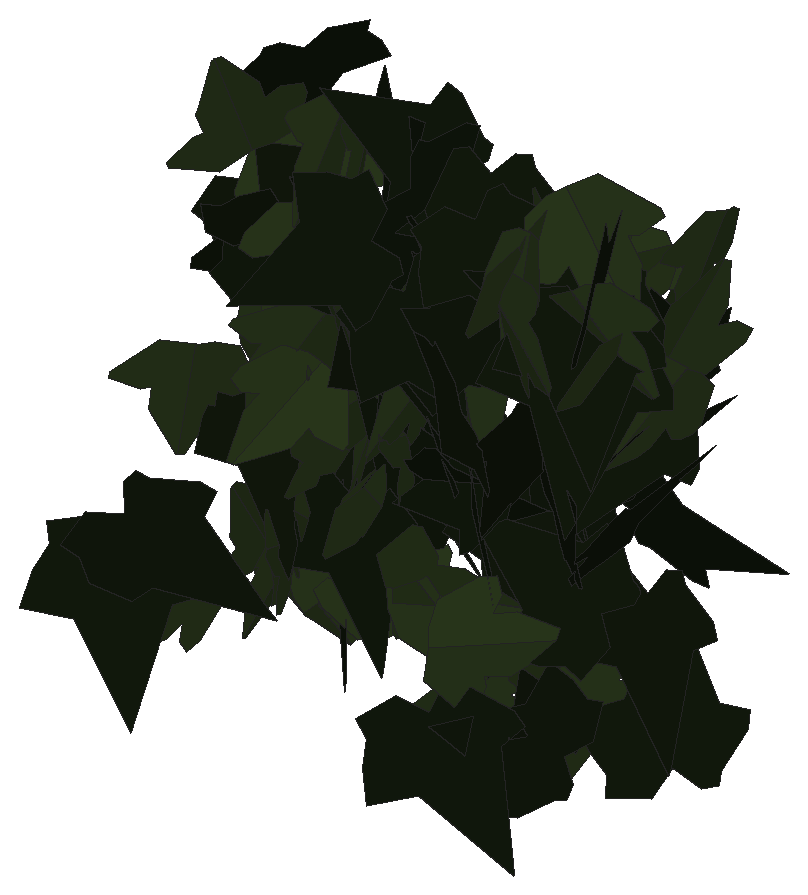
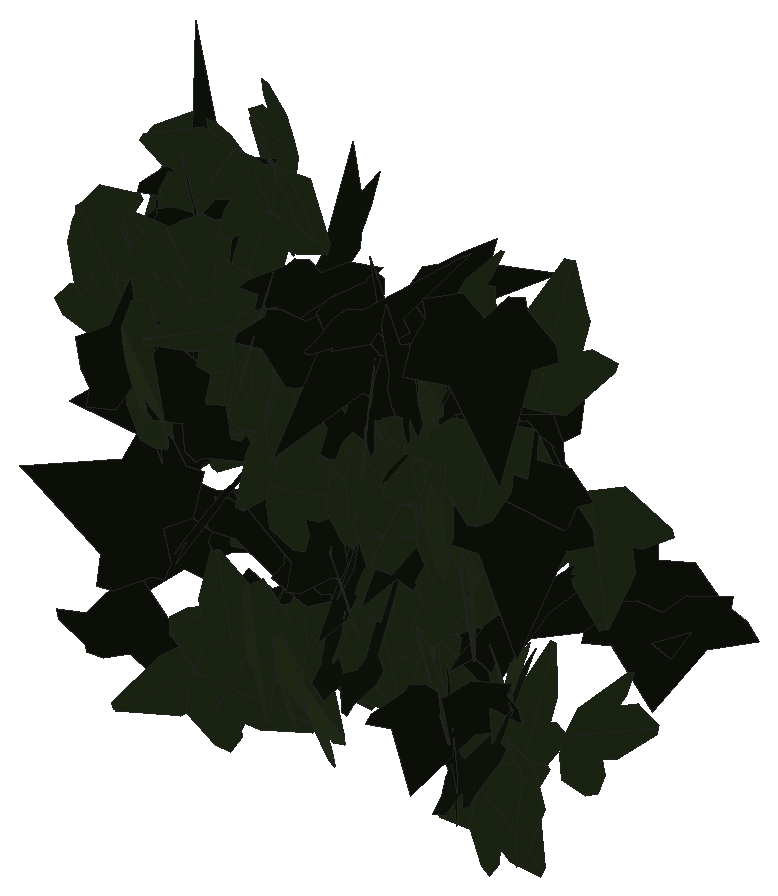
# SketchUp Ruby script. Lengths in inches.
U = 1.inch
M = Sketchup.active_model
def pt(a) = Geom::Point3d.new(a.map { |v| v * U })
def face(e, loops, mat)
  f = e.add_face(loops[0].map { |a| pt(a) })
  loops[1..].each { |l| e.add_face(l.map { |a| pt(a) }).erase! }
  f.material = f.back_material = mat if mat
  f
end
# faces: each face lists its corners as indices into pts; further lists are holes
def faces(e, pts, list, mat = nil) = list.each { |f| face(e, (f[0].is_a?(Array) ? f : [f]).map { |l| l.map { |i| pts[i] } }, mat) }
# xy, xz, yz: faces in a plane at the given z, y or x. An outline is a flat list of corners, or four numbers for a rectangle; further outlines are holes
def ring(l) = l.size == 4 ? [[l[0], l[1]], [l[2], l[1]], [l[2], l[3]], [l[0], l[3]]] : l.each_slice(2).to_a
def flat(e, list, mat, &to3) = list.each { |f| face(e, (f[0].is_a?(Array) ? f : [f]).map { |l| ring(l).map { |u, v| to3.(u, v) } }, mat) }
def xy(e, z, list, mat = nil) = flat(e, list, mat) { |x, y| [x, y, z] }
def xz(e, y, list, mat = nil) = flat(e, list, mat) { |x, z| [x, y, z] }
def yz(e, x, list, mat = nil) = flat(e, list, mat) { |y, z| [x, y, z] }
def lines(e, pts, list) = list.each { |a, b| e.add_line(pt(pts[a]), pt(pts[b])) }
# prism: a flat outline (further loops are holes) pulled along v
def prism(e, loops, v, mat = nil)
  f = face(e, loops, mat); d = Geom::Vector3d.new(v.map { |x| x * U })
  f.pushpull(f.normal.samedirection?(d) ? d.length : -d.length)
end
def box(e, o, s, mat = nil) = prism(e, [[o, [o[0] + s[0], o[1], o[2]], [o[0] + s[0], o[1] + s[1], o[2]], [o[0], o[1] + s[1], o[2]]]], [0, 0, s[2]], mat)
def at(x, y, z, deg = 0) = Geom::Transformation.translation(pt([x, y, z])) * Geom::Transformation.rotation(ORIGIN, Z_AXIS, deg.degrees)
def axes(o, x, y, z) = Geom::Transformation.new([*x, 0, *y, 0, *z, 0, *pt(o).to_a, 1])
def part(name) = M.definitions.add(name)
# library, detail: a bought-in or finely detailed component or shape, given as its bounding box
def library(name, o, s) = part(name).tap { |d| box(d.entities, o, s) }
def detail(e, o, s) = box(e.add_group.entities, o, s)
def put(e, d, t, mat = nil) = e.add_instance(d, t).tap { |i| i.material = mat if mat }
def group(e, t, mat = nil) = e.add_group.tap { |g| g.transformation = t; g.material = mat if mat }.entities
root = M.entities
M.materials.add("efeu1").color = [18, 25, 13]
M.materials.add("efeu2").color = [43, 57, 29]
c1 = part("ivyleaf_9")
p = [[1.54,2.16,1.25],[1.36,2.04,1.19],[-0.21,0.99,0.68],[-0.71,1.11,0.82],[-0.85,0.86,0.67],[-0.8,0.17,0.21],
  [-0.9,-0.01,0.1],[-0.67,-0.16,-0.02],[-0.08,-0.08,-0.05],[-0.03,-0.6,-0.4],[0.65,-0.88,-0.66],[0.83,-0.6,-0.49],
  [1.29,-0.42,-0.43],[1.8125,-0.07,-0.26],[1.21,0.44,0.15]]
faces(c1.entities,p,[[0,1,2,3,4,5,6,7,8,9,10,11,12,13,14]],"efeu1")
c2 = part("ivyleaf_10")
p = [[0,0.5,-0.03],[-0.0625,2.02,-0.43],[-0.19,2.01,-0.46],[-0.54,1.05,-0.29],[-0.52,0.625,-0.18],[-0.83,0.76,-0.28],
  [-1.16,0.64,-0.33],[-1.15,0.33,-0.24],[-0.77,-0.39,0.02],[-0.3,-0.51,0.16],[0.04,-0.48,0.23],[-0.02,2.01,-0.4375],
  [-0.06,2.01,-0.43],[0.04,-0.49,0.23],[0.67,-0.49,0.14],[1.38,0.36,-0.2],[1.375,0.51,-0.24],[0.81,0.65,-0.19],
  [0.62,0.59,-0.15],[0.6,1.09,-0.28],[0.5,1.23,-0.31]]
faces(c2.entities,p,[[0,1,2,3,4,5,6,7,8,9,10],[11,12,0,13,14,15,16,17,18,19,20]],"efeu2")
put(root,c1,axes([524.83,131.26,166.07],[-0.33768,-0.70628,-0.39631],[0.18411,0.35119,-0.78275],[0.78867,-0.38439,0.01304]))
put(root,c1,axes([530.67,131.73,170.2],[-0.07037,-0.33618,0.8001],[0.17324,-0.79201,-0.31754],[0.85039,0.13353,0.1309]))
put(root,c1,axes([525.15,131.12,166.79],[-0.00324,-0.09918,-0.87578],[0.39129,0.78459,-0.0903],[0.78976,-0.38914,0.04115]))
put(root,c2,axes([531.55,131.88,171.93],[-0.12147,0.13012,-0.78485],[0.54193,-0.56772,-0.17799],[-0.58244,-0.55537,-0.00193]))
put(root,c1,axes([530.2,131.6875,165.03],[-0.16384,-0.49695,-0.6787],[0.3544,0.58631,-0.51485],[0.76288,-0.3791,0.09342]))
put(root,c2,axes([530.38,131.99,166.21],[0.0291,-0.18103,-0.81104],[0.58754,0.57838,-0.10802],[0.58766,-0.5693,0.14816]))
put(root,c2,axes([524.8125,133.125,164.82],[-0.15719,-0.20614,0.77495],[0.12655,-0.78618,-0.18346],[0.79185,0.08473,0.18315]))
put(root,c1,axes([527.77,133.2,171.31],[-0.42129,-0.39468,0.56978],[-0.37791,-0.42814,-0.57599],[0.58103,-0.56464,0.03849]))
put(root,c1,axes([532.14,132.8125,171.72],[-0.38102,-0.63351,-0.36322],[0.22429,0.28837,-0.73823],[0.69495,-0.4404,0.03911]))
put(root,c1,axes([531.28,133.14,168.17],[-0.03344,-0.04847,0.86819],[0.28188,-0.82252,-0.03507],[0.82259,0.27988,0.04731]))
put(root,c2,axes([530.8125,132.92,172.19],[0.68256,-0.389,0.246],[0.21069,-0.12712,-0.7856],[0.4092,0.71431,-0.00584]))
put(root,c1,axes([531.3,133.21,164.18],[-0.08881,-0.05871,0.77051],[-0.61522,-0.46393,-0.10626],[0.46758,-0.62156,0.00653]))
put(root,c1,axes([532,133.07,171.17],[-0.54813,-0.70434,-0.32675],[0.20045,0.25805,-0.89249],[0.75012,-0.58363,-0.00027]))
put(root,c2,axes([532.25,132.74,171.99],[-0.66193,-0.01059,-0.40762],[0.40749,0.01078,-0.66201],[0.01466,-0.7773,-0.00363]))
put(root,c1,axes([531.94,133.12,171.56],[0.0001,0.50919,0.71944],[-0.06815,-0.71728,0.50767],[0.87876,-0.05568,0.03929]))
put(root,c2,axes([524.84,132.94,168.43],[-0.56624,-0.593,0.10866],[-0.06735,-0.08591,-0.81986],[0.5991,-0.57014,0.01053]))
put(root,c2,axes([532.52,132.99,171.28],[0.07296,-0.88071,-0.02433],[-0.00149,0.02429,-0.88373],[0.88104,0.07297,0.00052]))
put(root,c1,axes([531.25,132.96,169.81],[-0.09911,0.68835,-0.5205],[0.08396,-0.51374,-0.69541],[-0.85889,-0.12965,-0.00792]))
put(root,c2,axes([526.66,133.17,168.63],[0.51564,0.31871,-0.46657],[-0.39582,-0.24702,-0.60618],[-0.40322,0.65004,-0.0016]))
put(root,c1,axes([529.7,133.49,167.01],[-0.13232,0.06257,0.84388],[0.09722,-0.84735,0.07807],[0.84059,0.10785,0.1238]))
put(root,c2,axes([526.64,133.34,169.4],[-0.35373,-0.58412,0.4179],[-0.2198,-0.35544,-0.68287],[0.68375,-0.41644,-0.00333]))
put(root,c2,axes([528.72,133.08,165.93],[-0.14963,-0.09225,0.88799],[0.82092,0.33964,0.17361],[-0.35087,0.834,0.02751]))
put(root,c2,axes([527.73,132.95,169.95],[-0.02166,0.01381,0.77347],[-0.71103,0.30446,-0.02534],[-0.30475,-0.71135,0.00417]))
put(root,c2,axes([529.73,132.97,164.72],[-0.47195,-0.41579,-0.57038],[0.45046,0.35082,-0.62846],[0.54342,-0.65192,0.02559]))
put(root,c2,axes([529.01,133.25,165.9],[-0.6294,-0.14357,-0.40165],[0.40387,0.02971,-0.6435],[0.13721,-0.74605,0.05167]))
put(root,c1,axes([530.11,133.28,168.2],[-0.60442,0.37288,0.29163],[-0.24716,0.1548,-0.71018],[-0.40373,-0.653,-0.00182]))
put(root,c2,axes([526.48,133.5,170.88],[0.57668,0.38275,-0.24351],[-0.20508,-0.13135,-0.69213],[-0.40465,0.61205,0.00375]))
put(root,c2,axes([525.72,133.89,165.36],[-0.36296,0.24349,0.72411],[0.49871,-0.53178,0.42879],[0.57872,0.61097,0.08463]))
put(root,c2,axes([528.16,134.09,168.91],[-0.0036,-0.27996,0.77289],[0.25579,-0.73491,-0.26501],[0.78122,0.23933,0.09033]))
put(root,c1,axes([532.14,132.97,167.89],[-0.10416,0.73094,-0.26665],[-0.03631,0.26417,0.73832],[0.77721,0.1103,-0.00124]))
put(root,c1,axes([531.5,133.83,171.625],[-0.46135,-0.61749,-0.21894],[0.13553,0.17203,-0.77078],[0.64098,-0.48081,0.00539]))
put(root,c2,axes([525.33,133.77,168.81],[-0.05503,0.04318,-0.72069],[0.6025,-0.39551,-0.06971],[-0.39781,-0.60498,-0.00587]))
put(root,c1,axes([531.53,133.74,166.39],[-0.56293,-0.4876,-0.29346],[-0.19672,-0.22061,0.7439],[-0.53402,0.59526,0.03531]))
put(root,c1,axes([528.83,133.59,167.47],[0.55109,0.18256,-0.49055],[0.45821,0.17604,0.58028],[0.253,-0.71649,0.01758]))
put(root,c2,axes([530.61,133.29,171.99],[-0.19029,-0.7711,-0.50217],[0.13692,0.48336,-0.7941],[0.90996,-0.23398,0.01447]))
put(root,c1,axes([527.1875,134.3,169.17],[0.45596,-0.43502,-0.60219],[0.43981,-0.41136,0.63018],[-0.5987,-0.63349,0.00432]))
put(root,c2,axes([527.77,134.14,167.73],[-0.37409,0.23327,0.68753],[0.41937,-0.56192,0.41884],[0.59265,0.54487,0.1376]))
put(root,c2,axes([529.6,134.08,165.1],[0.27593,-0.73905,0.40423],[0.18018,-0.36374,-0.78801],[0.82288,0.32747,0.037]))
put(root,c1,axes([527.06,133.84,166.47],[-0.45072,-0.26509,-0.65886],[0.59257,0.28975,-0.52194],[0.39145,-0.74384,0.03149]))
put(root,c2,axes([526.52,134.19,167.12],[-0.24711,-0.41663,-0.55415],[-0.18121,-0.52903,0.47855],[-0.66919,0.2971,0.07504]))
put(root,c1,axes([528.28,133.55,170.42],[0.15786,-0.60152,-0.6506],[0.00209,0.6611,-0.61071],[0.88606,0.10561,0.11735]))
put(root,c2,axes([526.24,134.26,172.05],[-0.0504,-0.3943,0.64119],[0.3434,-0.5839,-0.33207],[0.66983,0.26967,0.21849]))
put(root,c1,axes([527.46,133.8,170.01],[0.4582,-0.61319,-0.18487],[-0.09026,0.16321,-0.76508],[0.63406,0.46635,0.02468]))
put(root,c1,axes([530.28,134.46,164.72],[-0.05622,-0.46218,0.69257],[-0.01843,-0.69328,-0.46416],[0.83242,-0.04656,0.0365]))
put(root,c2,axes([532.48,134.2,170.14],[-0.30347,-0.61715,0.51894],[-0.17618,-0.49033,-0.68615],[0.78685,-0.34781,0.04651]))
put(root,c1,axes([525.62,133.7,169.44],[-0.36122,0.19357,0.67789],[0.61601,-0.28376,0.40927],[0.34284,0.71379,-0.02114]))
put(root,c1,axes([528.77,133.57,170.33],[0.11288,-0.084,-0.88602],[0.54432,0.71312,0.00174],[0.70414,-0.5378,0.14069]))
put(root,c2,axes([525.53,134.23,165.81],[0.14512,-0.18933,-0.69325],[0.42317,-0.54911,0.23855],[-0.58084,-0.44736,0.00059]))
put(root,c2,axes([525.07,134.29,165.15],[-0.07185,-0.58739,-0.48252],[-0.07828,-0.47638,0.59157],[-0.75612,0.10513,-0.01539]))
put(root,c1,axes([530.13,134.21,167.18],[-0.66324,-0.38951,-0.27534],[0.23739,0.1395,-0.76916],[0.41373,-0.70445,-0.00007]))
put(root,c1,axes([525.21,134.24,167.31],[0.06167,-0.85524,-0.10599],[-0.0086,0.10565,-0.85746],[0.86174,0.06226,-0.00097]))
put(root,c2,axes([529.38,133.71,168.76],[0.62823,-0.18605,0.63949],[-0.61202,0.18541,0.65519],[-0.26265,-0.87706,0.00285]))
put(root,c2,axes([524.73,134.33,171.5],[-0.44943,-0.66729,-0.36218],[-0.15262,-0.33288,0.80271],[-0.74375,0.47154,0.05413]))
put(root,c1,axes([532.03,134.48,169.54],[-0.43571,-0.62066,0.17912],[-0.09604,-0.15142,-0.75829],[0.63881,-0.4461,0.00817]))
put(root,c2,axes([531.15,133.8125,172.63],[0.65344,0.38111,0.45401],[0.36578,0.27249,-0.75519],[-0.46645,0.74757,0.04381]))
put(root,c1,axes([532.13,134.18,166.55],[-0.48026,-0.30528,-0.63224],[0.56166,0.29255,-0.56791],[0.42126,-0.7381,0.0364]))
put(root,c1,axes([525.04,133.81,170.02],[0.38783,0.00681,0.67598],[0.676,-0.00902,-0.38775],[0.00443,0.77928,-0.0104]))
put(root,c2,axes([527.46,133.78,166.79],[-0.27705,-0.58567,-0.44141],[0.20692,0.39027,-0.64768],[0.70359,-0.34539,0.01666]))
put(root,c2,axes([527.76,133.59,169.87],[0.03386,-0.15486,-0.73455],[-0.28243,0.67865,-0.15609],[0.69554,0.28311,-0.02762]))
put(root,c2,axes([527.5,134.06,164.93],[0.61022,0.41697,0.37283],[-0.34348,-0.15614,0.7368],[0.44146,-0.69785,0.05791]))
put(root,c2,axes([530.72,134.17,164.79],[-0.35483,-0.63538,0.01556],[0.0171,0.00827,0.72766],[-0.63534,0.35507,0.0109]))
put(root,c1,axes([527.91,134.65,167.9],[0.52799,-0.20839,-0.71065],[0.66847,-0.24155,0.56748],[-0.31876,-0.85174,0.01293]))
put(root,c2,axes([528,133.78,169.92],[-0.15583,-0.59672,-0.59249],[0.21352,0.55475,-0.61487],[0.81335,-0.25996,0.0479]))
put(root,c1,axes([529.08,134.14,171.625],[0.02752,-0.56762,-0.51326],[0.19473,0.50188,-0.54459],[0.74007,-0.11095,0.16239]))
put(root,c1,axes([528.41,134.37,166.57],[0.39343,0.01244,0.76483],[-0.758,0.12186,0.38793],[-0.10274,-0.85142,0.06669]))
put(root,c2,axes([530.26,134.43,168.95],[0.66464,-0.04026,0.50054],[0.49927,-0.036,-0.66585],[0.05381,0.83126,-0.00459]))
put(root,c2,axes([525.81,134.4375,165.33],[0.38061,-0.01616,0.7818],[0.78196,0.01005,-0.38049],[-0.00196,0.86947,0.01892]))
put(root,c2,axes([528.57,134.85,165.01],[0.39373,-0.49896,0.51455],[0.29527,-0.42203,-0.63518],[0.6531,0.49161,-0.02304]))
put(root,c2,axes([531.61,134.74,168.49],[0.07625,-0.6073,-0.35431],[0.12715,-0.3386,0.60773],[-0.69151,-0.12923,0.07268]))
put(root,c1,axes([531.66,133.83,168.49],[-0.11203,0.64599,-0.46863],[-0.07738,0.46221,0.65563],[0.79431,0.13613,-0.00223]))
put(root,c1,axes([532.54,134.23,164.08],[-0.83985,-0.05646,0.23177],[0.23138,0.01359,0.84174],[-0.05804,0.87114,0.00189]))
put(root,c1,axes([526.02,134.82,165.45],[-0.20499,0.04915,-0.84771],[0.82516,-0.19423,-0.2108],[-0.20035,-0.85024,-0.00085]))
put(root,c2,axes([530.9375,133.95,164.52],[-0.22302,-0.224,-0.88221],[0.56968,0.67406,-0.31516],[0.70989,-0.6113,-0.02425]))
put(root,c1,axes([526.46,134.85,170.39],[0.36032,-0.65111,0.19844],[0.09538,-0.17402,-0.74416],[0.67397,0.37273,-0.00078]))
put(root,c1,axes([527.05,135.23,168.28],[-0.01567,-0.43981,0.68525],[0.01116,-0.68543,-0.43967],[0.81417,0.00093,0.01922]))
put(root,c1,axes([527.54,134.82,170.07],[0.2286,-0.2623,0.67593],[0.5364,-0.41565,-0.34271],[0.48781,0.57998,0.06009]))
put(root,c2,axes([527.4,134.76,166.76],[-0.2175,-0.75893,0.10008],[-0.0113,-0.10085,-0.7893],[0.76542,-0.21714,0.01679]))
put(root,c1,axes([525.9,134.84,170.08],[0.25246,-0.22291,0.73659],[0.5885,-0.44362,-0.33595],[0.49591,0.63992,0.02368]))
put(root,c2,axes([524.98,134.68,164.68],[-0.51757,0.14037,-0.65553],[0.6277,-0.18934,-0.53614],[-0.23541,-0.81348,0.01168]))
put(root,c2,axes([529.82,134.6,170.37],[-0.68247,-0.2581,-0.08969],[0.08299,0.03413,-0.72964],[0.26033,-0.68749,-0.00255]))
put(root,c2,axes([531.27,134.8125,171.73],[0.43441,0.50582,-0.23347],[-0.168,-0.16333,-0.66646],[-0.53116,0.46534,0.01985]))
put(root,c2,axes([531.19,134.65,170.85],[-0.48192,-0.35196,0.41518],[0.33039,0.25151,0.59672],[-0.43253,0.58426,-0.00677]))
put(root,c1,axes([530.125,134.91,168.02],[0.36787,-0.7401,-0.13066],[-0.05863,0.11677,-0.82649],[0.74925,0.37252,-0.00052]))
put(root,c2,axes([527.82,134.39,170.3],[0.20896,-0.41407,-0.59617],[-0.14885,0.58276,-0.45692],[0.71043,0.24389,0.07962]))
put(root,c2,axes([532.2,134.74,170.36],[-0.26557,-0.77695,0.23113],[0.11959,0.203,0.81981],[-0.80173,0.28764,0.04573]))
put(root,c2,axes([527.92,135.03,167.4],[0.45747,-0.57077,0.20846],[0.12773,-0.16478,-0.73147],[0.59407,0.47496,-0.00325]))
put(root,c2,axes([524.88,135.16,164.53],[0.02648,-0.64237,0.38785],[0.02037,-0.38733,-0.6429],[0.7501,0.0332,0.00377]))
put(root,c1,axes([528.01,134.99,168.02],[0.45245,-0.37743,0.57126],[0.47938,-0.31426,-0.58731],[0.48885,0.65749,0.04721]))
put(root,c2,axes([526.09,134.48,167.72],[-0.15849,-0.47046,-0.53826],[0.23653,0.48577,-0.49423],[0.67462,-0.28084,0.04683]))
put(root,c1,axes([530.93,134.93,168.875],[0.12757,-0.05148,0.74925],[-0.71923,0.21037,0.13692],[-0.21617,-0.73034,-0.01337]))
put(root,c2,axes([530.2,135.125,164.7],[-0.18735,-0.13027,0.72521],[-0.56172,-0.45899,-0.22757],[0.47682,-0.5919,0.01686]))
put(root,c1,axes([527.07,134.6,168.53],[0.81194,-0.0685,-0.22433],[-0.22334,0.02115,-0.81482],[0.07166,0.84209,0.00222]))
put(root,c1,axes([525.35,135.31,164.78],[0.45987,-0.63846,-0.0692],[0.04695,-0.05147,0.78679],[-0.64048,-0.46219,0.00798]))
put(root,c2,axes([529.39,135.3,170.59],[-0.23213,0.28947,0.71111],[0.45637,-0.54538,0.37099],[0.61741,0.51197,-0.00686]))
put(root,c1,axes([524.78,134.63,169.54],[0.43307,0.58831,-0.33978],[-0.21158,-0.26612,-0.73043],[-0.6456,0.48186,0.01145]))
put(root,c2,axes([527.5,135.29,169.13],[-0.02833,-0.49828,0.49008],[-0.04097,-0.48845,-0.499],[0.6977,-0.04892,-0.0094]))
put(root,c2,axes([529.72,134.89,170.42],[-0.54888,0.23511,-0.41374],[0.38216,-0.15857,-0.5971],[-0.28356,-0.66881,-0.00387]))
put(root,c2,axes([528.97,134.91,170.1],[-0.66984,-0.4833,0.09558],[-0.06964,-0.06682,-0.82588],[0.48771,-0.67332,0.01335]))
put(root,c2,axes([526.4375,135.1,169.94],[-0.23436,-0.09509,0.77883],[0.77577,-0.1498,0.21515],[0.11749,0.79941,0.13295]))
put(root,c2,axes([525.81,134.79,168.25],[0.34437,-0.55506,-0.34467],[-0.15212,0.31079,-0.6525],[0.63541,0.37523,0.03059]))
put(root,c2,axes([526.98,135.22,168.48],[-0.14303,-0.0674,-0.69603],[-0.64592,-0.25949,0.15786],[-0.26795,0.6615,-0.00899]))
put(root,c1,axes([524.48,134.81,170.38],[0.07628,-0.23519,-0.81969],[0.55941,0.63495,-0.13012],[0.64364,-0.52398,0.21024]))
put(root,c1,axes([527.6875,135.36,171.49],[-0.20426,-0.77888,-0.18429],[-0.04707,-0.17818,0.80522],[-0.799,0.20962,-0.00033]))
put(root,c1,axes([527.73,135.22,165.72],[0.4273,-0.59077,0.26814],[-0.14865,0.22339,0.72904],[-0.63152,-0.45231,0.00983]))
put(root,c2,axes([525.7,135.36,169.46],[0.19589,-0.70049,0.35531],[0.12455,-0.33386,-0.72687],[0.77551,0.23056,0.02699]))
put(root,c1,axes([531.72,135.22,169.45],[0.25397,0.44224,0.57746],[-0.3991,-0.42661,0.50225],[0.60807,-0.46472,0.08846]))
put(root,c2,axes([528.91,134.75,169.66],[-0.47276,-0.514,-0.45629],[0.29562,0.34791,-0.69819],[0.62049,-0.55738,-0.01502]))
put(root,c2,axes([530.04,134.5625,170.69],[0.00652,0.04546,0.77785],[0.37341,0.68255,-0.04302],[-0.68387,0.37313,-0.01607]))
put(root,c2,axes([529.5625,135.01,166.1],[0.25055,-0.72504,-0.19623],[-0.05948,0.18705,-0.76709],[0.74876,0.25747,0.00472]))
put(root,c2,axes([525.94,135.46,171.48],[0.19104,-0.44079,0.55727],[0.37467,-0.42782,-0.46684],[0.60371,0.40499,0.11338]))
put(root,c1,axes([527.67,134.46,171.55],[0.07276,-0.05628,-0.90504],[-0.40135,0.81218,-0.08277],[0.81314,0.40591,0.04013]))
put(root,c2,axes([525.91,135.35,168.79],[-0.36218,0.10231,0.74224],[0.7168,-0.19271,0.37632],[0.21814,0.80309,-0.00425]))
put(root,c2,axes([528.4,135.68,168.89],[0.0421,-0.3302,0.6621],[0.08574,-0.65653,-0.33287],[0.73489,0.09552,0.0009]))
put(root,c1,axes([528.33,135.34,171.57],[-0.35349,-0.59308,-0.37565],[0.21868,0.30664,-0.6899],[0.66712,-0.41478,0.0271]))
put(root,c2,axes([527.26,135.3,168.99],[-0.54716,-0.09519,-0.47966],[-0.47446,-0.07095,0.55531],[-0.1184,0.72417,-0.00864]))
put(root,c1,axes([531.24,135.26,167.12],[0.45394,-0.25146,0.74257],[0.66904,-0.32306,-0.51839],[0.4087,0.80815,0.02383]))
put(root,c2,axes([526.05,135.22,169.96],[-0.39164,0.08832,-0.63245],[0.61062,-0.16536,-0.40122],[-0.18691,-0.72528,0.01446]))
put(root,c2,axes([526.14,135.27,166.86],[0.48669,-0.55424,-0.11932],[-0.07893,0.08948,-0.73759],[0.56141,0.49305,-0.00027]))
put(root,c1,axes([526.28,135.53,170.9375],[-0.06237,0.22349,0.79023],[0.26629,-0.74418,0.23148],[0.77685,0.27304,-0.0159]))
put(root,c1,axes([525.7,135.35,166.13],[-0.20519,-0.63441,-0.45047],[0.1484,0.42541,-0.66672],[0.76379,-0.25309,0.00853]))
put(root,c2,axes([532.21,135.59,171.98],[0.07174,-0.71504,0.26849],[0.05836,-0.26375,-0.71801],[0.76155,0.08757,0.02973]))
put(root,c2,axes([524.93,135.3125,170.75],[0.67666,0.5304,0.11601],[0.08785,0.07596,-0.85974],[-0.53578,0.68231,0.00554]))
put(root,c2,axes([527.26,134.98,167.57],[0.13524,-0.45684,-0.57237],[0.11053,0.58812,-0.44329],[0.72395,-0.00445,0.17461]))
put(root,c1,axes([525.1,135.16,172.63],[0.16101,0.74686,-0.28948],[-0.06066,-0.28305,-0.76402],[-0.7987,0.17206,-0.00033]))
put(root,c2,axes([531.3,135.71,170.34],[0.3597,-0.63942,0.30907],[0.1569,-0.26634,-0.73363],[0.69265,0.39239,0.00568]))
